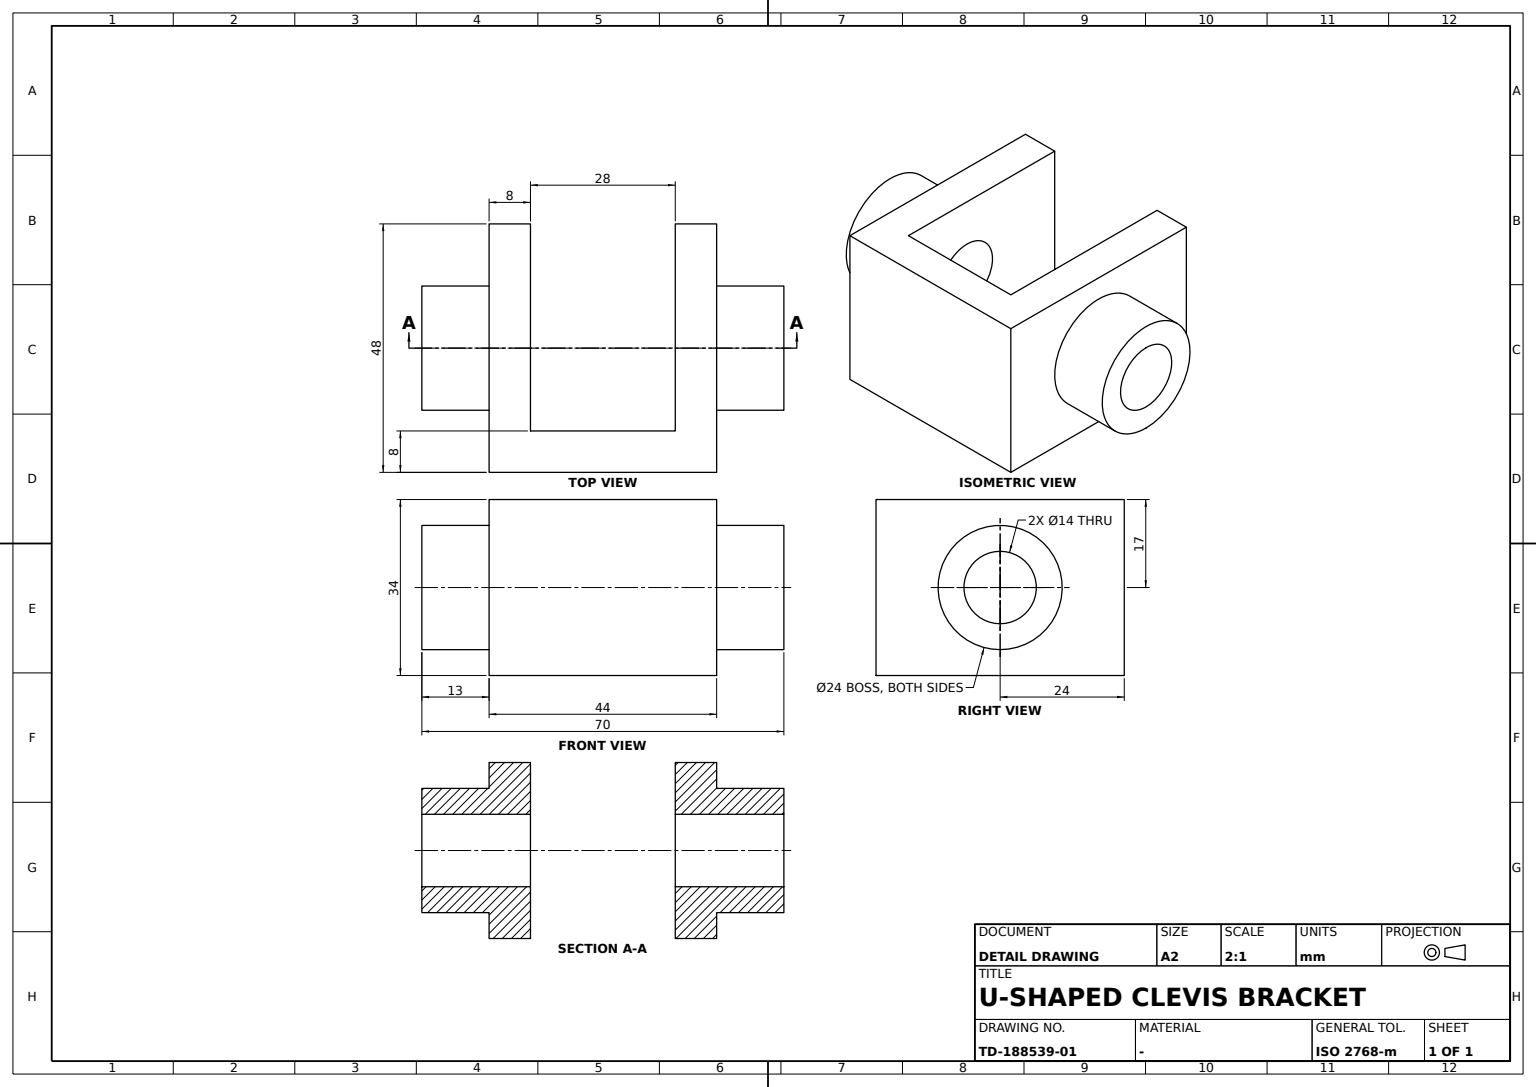
ISO-10303-21;
HEADER;
FILE_DESCRIPTION((''),'2;1');
FILE_NAME('','',(''),(''),'','','');
FILE_SCHEMA(('AUTOMOTIVE_DESIGN'));
ENDSEC;
DATA;
#1=APPLICATION_CONTEXT('');
#2=PRODUCT_CONTEXT('',#1,'mechanical');
#3=PRODUCT('','','',(#2));
#4=PRODUCT_DEFINITION_FORMATION('','',#3);
#5=PRODUCT_DEFINITION_CONTEXT('',#1,'design');
#6=PRODUCT_DEFINITION('','',#4,#5);
#7=PRODUCT_DEFINITION_SHAPE('','',#6);
#8=(LENGTH_UNIT()NAMED_UNIT(*)SI_UNIT(.MILLI.,.METRE.));
#9=(NAMED_UNIT(*)PLANE_ANGLE_UNIT()SI_UNIT($,.RADIAN.));
#10=(NAMED_UNIT(*)SI_UNIT($,.STERADIAN.)SOLID_ANGLE_UNIT());
#11=UNCERTAINTY_MEASURE_WITH_UNIT(LENGTH_MEASURE(0.005),#8,'distance_accuracy_value','');
#12=(GEOMETRIC_REPRESENTATION_CONTEXT(3)GLOBAL_UNCERTAINTY_ASSIGNED_CONTEXT((#11))GLOBAL_UNIT_ASSIGNED_CONTEXT((#8,#9,#10))REPRESENTATION_CONTEXT('',''));
#13=CARTESIAN_POINT('',(-35.,0.,5.));
#14=VERTEX_POINT('',#13);
#15=CARTESIAN_POINT('',(-35.,0.,17.));
#16=DIRECTION('',(1.,0.,0.));
#17=DIRECTION('',(0.,0.,-1.));
#18=AXIS2_PLACEMENT_3D('',#15,#16,#17);
#19=CIRCLE('',#18,12.);
#20=EDGE_CURVE('',#14,#14,#19,.T.);
#21=ORIENTED_EDGE('',*,*,#20,.F.);
#22=EDGE_LOOP('',(#21));
#23=FACE_BOUND('',#22,.T.);
#24=CARTESIAN_POINT('',(-35.,0.,10.));
#25=VERTEX_POINT('',#24);
#26=CIRCLE('',#18,7.);
#27=EDGE_CURVE('',#25,#25,#26,.T.);
#28=ORIENTED_EDGE('',*,*,#27,.T.);
#29=EDGE_LOOP('',(#28));
#30=FACE_BOUND('',#29,.T.);
#31=CARTESIAN_POINT('',(-35.,0.,0.));
#32=DIRECTION('',(0.,1.,0.));
#33=AXIS2_PLACEMENT_3D('',#31,#16,#32);
#34=PLANE('',#33);
#35=ADVANCED_FACE('',(#23,#30),#34,.F.);
#36=CARTESIAN_POINT('',(14.,0.,24.));
#37=VERTEX_POINT('',#36);
#38=CARTESIAN_POINT('',(14.,0.,17.));
#39=DIRECTION('',(-1.,0.,0.));
#40=DIRECTION('',(0.,0.,1.));
#41=AXIS2_PLACEMENT_3D('',#38,#39,#40);
#42=CIRCLE('',#41,7.);
#43=EDGE_CURVE('',#37,#37,#42,.T.);
#44=ORIENTED_EDGE('',*,*,#43,.T.);
#45=EDGE_LOOP('',(#44));
#46=FACE_BOUND('',#45,.T.);
#47=CARTESIAN_POINT('',(35.,0.,10.));
#48=VERTEX_POINT('',#47);
#49=CARTESIAN_POINT('',(35.,0.,17.));
#50=AXIS2_PLACEMENT_3D('',#49,#16,#17);
#51=CIRCLE('',#50,7.);
#52=EDGE_CURVE('',#48,#48,#51,.T.);
#53=ORIENTED_EDGE('',*,*,#52,.T.);
#54=EDGE_LOOP('',(#53));
#55=FACE_BOUND('',#54,.T.);
#56=CARTESIAN_POINT('',(20.5,0.,17.));
#57=DIRECTION('',(0.,-1.,0.));
#58=AXIS2_PLACEMENT_3D('',#56,#39,#57);
#59=CYLINDRICAL_SURFACE('',#58,7.);
#60=ADVANCED_FACE('',(#46,#55),#59,.F.);
#61=CARTESIAN_POINT('',(-22.,24.,0.));
#62=VERTEX_POINT('',#61);
#63=CARTESIAN_POINT('',(-22.,24.,34.));
#64=VERTEX_POINT('',#63);
#65=VECTOR('',#40,1000.);
#66=LINE('',#61,#65);
#67=EDGE_CURVE('',#62,#64,#66,.T.);
#68=ORIENTED_EDGE('',*,*,#67,.T.);
#69=CARTESIAN_POINT('',(-14.,24.,34.));
#70=VERTEX_POINT('',#69);
#71=CARTESIAN_POINT('',(0.,24.,34.));
#72=VECTOR('',#39,1000.);
#73=LINE('',#71,#72);
#74=EDGE_CURVE('',#70,#64,#73,.T.);
#75=ORIENTED_EDGE('',*,*,#74,.F.);
#76=CARTESIAN_POINT('',(-14.,24.,0.));
#77=VERTEX_POINT('',#76);
#78=LINE('',#76,#65);
#79=EDGE_CURVE('',#77,#70,#78,.T.);
#80=ORIENTED_EDGE('',*,*,#79,.F.);
#81=CARTESIAN_POINT('',(0.,24.,0.));
#82=LINE('',#81,#72);
#83=EDGE_CURVE('',#77,#62,#82,.T.);
#84=ORIENTED_EDGE('',*,*,#83,.T.);
#85=EDGE_LOOP('',(#68,#75,#80,#84));
#86=FACE_BOUND('',#85,.T.);
#87=CARTESIAN_POINT('',(22.,24.,0.));
#88=AXIS2_PLACEMENT_3D('',#87,#32,#39);
#89=PLANE('',#88);
#90=ADVANCED_FACE('',(#86),#89,.T.);
#91=CARTESIAN_POINT('',(-22.,0.,29.));
#92=VERTEX_POINT('',#91);
#93=CARTESIAN_POINT('',(-22.,0.,17.));
#94=AXIS2_PLACEMENT_3D('',#93,#39,#40);
#95=CIRCLE('',#94,12.);
#96=EDGE_CURVE('',#92,#92,#95,.F.);
#97=ORIENTED_EDGE('',*,*,#96,.T.);
#98=EDGE_LOOP('',(#97));
#99=FACE_BOUND('',#98,.T.);
#100=CARTESIAN_POINT('',(-22.,-24.,34.));
#101=VERTEX_POINT('',#100);
#102=CARTESIAN_POINT('',(-22.,0.,34.));
#103=VECTOR('',#57,1000.);
#104=LINE('',#102,#103);
#105=EDGE_CURVE('',#64,#101,#104,.T.);
#106=ORIENTED_EDGE('',*,*,#105,.F.);
#107=ORIENTED_EDGE('',*,*,#67,.F.);
#108=CARTESIAN_POINT('',(-22.,-24.,0.));
#109=VERTEX_POINT('',#108);
#110=CARTESIAN_POINT('',(-22.,0.,0.));
#111=LINE('',#110,#103);
#112=EDGE_CURVE('',#62,#109,#111,.T.);
#113=ORIENTED_EDGE('',*,*,#112,.T.);
#114=LINE('',#108,#65);
#115=EDGE_CURVE('',#109,#101,#114,.T.);
#116=ORIENTED_EDGE('',*,*,#115,.T.);
#117=EDGE_LOOP('',(#106,#107,#113,#116));
#118=FACE_BOUND('',#117,.T.);
#119=AXIS2_PLACEMENT_3D('',#61,#39,#57);
#120=PLANE('',#119);
#121=ADVANCED_FACE('',(#99,#118),#120,.T.);
#122=ORIENTED_EDGE('',*,*,#96,.F.);
#123=EDGE_LOOP('',(#122));
#124=FACE_BOUND('',#123,.T.);
#125=ORIENTED_EDGE('',*,*,#20,.T.);
#126=EDGE_LOOP('',(#125));
#127=FACE_BOUND('',#126,.T.);
#128=CARTESIAN_POINT('',(28.5,0.,17.));
#129=AXIS2_PLACEMENT_3D('',#128,#16,#32);
#130=CYLINDRICAL_SURFACE('',#129,12.);
#131=ADVANCED_FACE('',(#124,#127),#130,.T.);
#132=VERTEX_POINT('',#87);
#133=CARTESIAN_POINT('',(14.,24.,0.));
#134=VERTEX_POINT('',#133);
#135=EDGE_CURVE('',#132,#134,#82,.T.);
#136=ORIENTED_EDGE('',*,*,#135,.F.);
#137=CARTESIAN_POINT('',(22.,-24.,0.));
#138=VERTEX_POINT('',#137);
#139=CARTESIAN_POINT('',(22.,0.,0.));
#140=VECTOR('',#32,1000.);
#141=LINE('',#139,#140);
#142=EDGE_CURVE('',#138,#132,#141,.T.);
#143=ORIENTED_EDGE('',*,*,#142,.F.);
#144=CARTESIAN_POINT('',(0.,-24.,0.));
#145=VECTOR('',#16,1000.);
#146=LINE('',#144,#145);
#147=EDGE_CURVE('',#109,#138,#146,.T.);
#148=ORIENTED_EDGE('',*,*,#147,.F.);
#149=ORIENTED_EDGE('',*,*,#112,.F.);
#150=ORIENTED_EDGE('',*,*,#83,.F.);
#151=CARTESIAN_POINT('',(-14.,-16.,0.));
#152=VERTEX_POINT('',#151);
#153=CARTESIAN_POINT('',(-14.,0.,0.));
#154=LINE('',#153,#140);
#155=EDGE_CURVE('',#152,#77,#154,.T.);
#156=ORIENTED_EDGE('',*,*,#155,.F.);
#157=CARTESIAN_POINT('',(14.,-16.,0.));
#158=VERTEX_POINT('',#157);
#159=CARTESIAN_POINT('',(0.,-16.,0.));
#160=LINE('',#159,#72);
#161=EDGE_CURVE('',#158,#152,#160,.T.);
#162=ORIENTED_EDGE('',*,*,#161,.F.);
#163=CARTESIAN_POINT('',(14.,0.,0.));
#164=LINE('',#163,#103);
#165=EDGE_CURVE('',#134,#158,#164,.T.);
#166=ORIENTED_EDGE('',*,*,#165,.F.);
#167=EDGE_LOOP('',(#136,#143,#148,#149,#150,#156,#162,#166));
#168=FACE_BOUND('',#167,.T.);
#169=CARTESIAN_POINT('',(0.,0.,0.));
#170=AXIS2_PLACEMENT_3D('',#169,#40,#16);
#171=PLANE('',#170);
#172=ADVANCED_FACE('',(#168),#171,.F.);
#173=ORIENTED_EDGE('',*,*,#147,.T.);
#174=CARTESIAN_POINT('',(22.,-24.,34.));
#175=VERTEX_POINT('',#174);
#176=LINE('',#137,#65);
#177=EDGE_CURVE('',#138,#175,#176,.T.);
#178=ORIENTED_EDGE('',*,*,#177,.T.);
#179=CARTESIAN_POINT('',(0.,-24.,34.));
#180=LINE('',#179,#145);
#181=EDGE_CURVE('',#101,#175,#180,.T.);
#182=ORIENTED_EDGE('',*,*,#181,.F.);
#183=ORIENTED_EDGE('',*,*,#115,.F.);
#184=EDGE_LOOP('',(#173,#178,#182,#183));
#185=FACE_BOUND('',#184,.T.);
#186=AXIS2_PLACEMENT_3D('',#108,#57,#16);
#187=PLANE('',#186);
#188=ADVANCED_FACE('',(#185),#187,.T.);
#189=CARTESIAN_POINT('',(35.,0.,5.));
#190=VERTEX_POINT('',#189);
#191=CIRCLE('',#50,12.);
#192=EDGE_CURVE('',#190,#190,#191,.T.);
#193=ORIENTED_EDGE('',*,*,#192,.T.);
#194=EDGE_LOOP('',(#193));
#195=FACE_BOUND('',#194,.T.);
#196=ORIENTED_EDGE('',*,*,#52,.F.);
#197=EDGE_LOOP('',(#196));
#198=FACE_BOUND('',#197,.T.);
#199=CARTESIAN_POINT('',(35.,0.,0.));
#200=AXIS2_PLACEMENT_3D('',#199,#16,#32);
#201=PLANE('',#200);
#202=ADVANCED_FACE('',(#195,#198),#201,.T.);
#203=CARTESIAN_POINT('',(-14.,-16.,34.));
#204=VERTEX_POINT('',#203);
#205=CARTESIAN_POINT('',(-14.,0.,34.));
#206=LINE('',#205,#140);
#207=EDGE_CURVE('',#204,#70,#206,.T.);
#208=ORIENTED_EDGE('',*,*,#207,.T.);
#209=ORIENTED_EDGE('',*,*,#74,.T.);
#210=ORIENTED_EDGE('',*,*,#105,.T.);
#211=ORIENTED_EDGE('',*,*,#181,.T.);
#212=CARTESIAN_POINT('',(22.,24.,34.));
#213=VERTEX_POINT('',#212);
#214=CARTESIAN_POINT('',(22.,0.,34.));
#215=LINE('',#214,#140);
#216=EDGE_CURVE('',#175,#213,#215,.T.);
#217=ORIENTED_EDGE('',*,*,#216,.T.);
#218=CARTESIAN_POINT('',(14.,24.,34.));
#219=VERTEX_POINT('',#218);
#220=EDGE_CURVE('',#213,#219,#73,.T.);
#221=ORIENTED_EDGE('',*,*,#220,.T.);
#222=CARTESIAN_POINT('',(14.,-16.,34.));
#223=VERTEX_POINT('',#222);
#224=CARTESIAN_POINT('',(14.,0.,34.));
#225=LINE('',#224,#103);
#226=EDGE_CURVE('',#219,#223,#225,.T.);
#227=ORIENTED_EDGE('',*,*,#226,.T.);
#228=CARTESIAN_POINT('',(0.,-16.,34.));
#229=LINE('',#228,#72);
#230=EDGE_CURVE('',#223,#204,#229,.T.);
#231=ORIENTED_EDGE('',*,*,#230,.T.);
#232=EDGE_LOOP('',(#208,#209,#210,#211,#217,#221,#227,#231));
#233=FACE_BOUND('',#232,.T.);
#234=CARTESIAN_POINT('',(0.,0.,34.));
#235=AXIS2_PLACEMENT_3D('',#234,#40,#16);
#236=PLANE('',#235);
#237=ADVANCED_FACE('',(#233),#236,.T.);
#238=LINE('',#151,#65);
#239=EDGE_CURVE('',#152,#204,#238,.T.);
#240=ORIENTED_EDGE('',*,*,#239,.T.);
#241=ORIENTED_EDGE('',*,*,#230,.F.);
#242=LINE('',#157,#65);
#243=EDGE_CURVE('',#158,#223,#242,.T.);
#244=ORIENTED_EDGE('',*,*,#243,.F.);
#245=ORIENTED_EDGE('',*,*,#161,.T.);
#246=EDGE_LOOP('',(#240,#241,#244,#245));
#247=FACE_BOUND('',#246,.T.);
#248=AXIS2_PLACEMENT_3D('',#157,#32,#39);
#249=PLANE('',#248);
#250=ADVANCED_FACE('',(#247),#249,.T.);
#251=ORIENTED_EDGE('',*,*,#239,.F.);
#252=ORIENTED_EDGE('',*,*,#155,.T.);
#253=ORIENTED_EDGE('',*,*,#79,.T.);
#254=ORIENTED_EDGE('',*,*,#207,.F.);
#255=EDGE_LOOP('',(#251,#252,#253,#254));
#256=FACE_BOUND('',#255,.T.);
#257=CARTESIAN_POINT('',(-14.,0.,10.));
#258=VERTEX_POINT('',#257);
#259=CARTESIAN_POINT('',(-14.,0.,17.));
#260=AXIS2_PLACEMENT_3D('',#259,#16,#17);
#261=CIRCLE('',#260,7.);
#262=EDGE_CURVE('',#258,#258,#261,.T.);
#263=ORIENTED_EDGE('',*,*,#262,.F.);
#264=EDGE_LOOP('',(#263));
#265=FACE_BOUND('',#264,.T.);
#266=AXIS2_PLACEMENT_3D('',#151,#16,#32);
#267=PLANE('',#266);
#268=ADVANCED_FACE('',(#256,#265),#267,.T.);
#269=LINE('',#133,#65);
#270=EDGE_CURVE('',#134,#219,#269,.T.);
#271=ORIENTED_EDGE('',*,*,#270,.T.);
#272=ORIENTED_EDGE('',*,*,#220,.F.);
#273=LINE('',#87,#65);
#274=EDGE_CURVE('',#132,#213,#273,.T.);
#275=ORIENTED_EDGE('',*,*,#274,.F.);
#276=ORIENTED_EDGE('',*,*,#135,.T.);
#277=EDGE_LOOP('',(#271,#272,#275,#276));
#278=FACE_BOUND('',#277,.T.);
#279=ADVANCED_FACE('',(#278),#89,.T.);
#280=ORIENTED_EDGE('',*,*,#192,.F.);
#281=EDGE_LOOP('',(#280));
#282=FACE_BOUND('',#281,.T.);
#283=CARTESIAN_POINT('',(22.,0.,5.));
#284=VERTEX_POINT('',#283);
#285=CARTESIAN_POINT('',(22.,0.,17.));
#286=AXIS2_PLACEMENT_3D('',#285,#16,#17);
#287=CIRCLE('',#286,12.);
#288=EDGE_CURVE('',#284,#284,#287,.T.);
#289=ORIENTED_EDGE('',*,*,#288,.T.);
#290=EDGE_LOOP('',(#289));
#291=FACE_BOUND('',#290,.T.);
#292=ADVANCED_FACE('',(#282,#291),#130,.T.);
#293=ORIENTED_EDGE('',*,*,#142,.T.);
#294=ORIENTED_EDGE('',*,*,#274,.T.);
#295=ORIENTED_EDGE('',*,*,#216,.F.);
#296=ORIENTED_EDGE('',*,*,#177,.F.);
#297=EDGE_LOOP('',(#293,#294,#295,#296));
#298=FACE_BOUND('',#297,.T.);
#299=ORIENTED_EDGE('',*,*,#288,.F.);
#300=EDGE_LOOP('',(#299));
#301=FACE_BOUND('',#300,.T.);
#302=AXIS2_PLACEMENT_3D('',#137,#16,#32);
#303=PLANE('',#302);
#304=ADVANCED_FACE('',(#298,#301),#303,.T.);
#305=ORIENTED_EDGE('',*,*,#262,.T.);
#306=EDGE_LOOP('',(#305));
#307=FACE_BOUND('',#306,.T.);
#308=ORIENTED_EDGE('',*,*,#27,.F.);
#309=EDGE_LOOP('',(#308));
#310=FACE_BOUND('',#309,.T.);
#311=ADVANCED_FACE('',(#307,#310),#59,.F.);
#312=ORIENTED_EDGE('',*,*,#226,.F.);
#313=ORIENTED_EDGE('',*,*,#270,.F.);
#314=ORIENTED_EDGE('',*,*,#165,.T.);
#315=ORIENTED_EDGE('',*,*,#243,.T.);
#316=EDGE_LOOP('',(#312,#313,#314,#315));
#317=FACE_BOUND('',#316,.T.);
#318=ORIENTED_EDGE('',*,*,#43,.F.);
#319=EDGE_LOOP('',(#318));
#320=FACE_BOUND('',#319,.T.);
#321=AXIS2_PLACEMENT_3D('',#133,#39,#57);
#322=PLANE('',#321);
#323=ADVANCED_FACE('',(#317,#320),#322,.T.);
#324=CLOSED_SHELL('',(#35,#60,#90,#121,#131,#172,#188,#202,#237,#250,#268,#279,#292,#304,#311,#323));
#325=MANIFOLD_SOLID_BREP('',#324);
#326=ADVANCED_BREP_SHAPE_REPRESENTATION('',(#325),#12);
#327=SHAPE_DEFINITION_REPRESENTATION(#7,#326);
ENDSEC;
END-ISO-10303-21;
